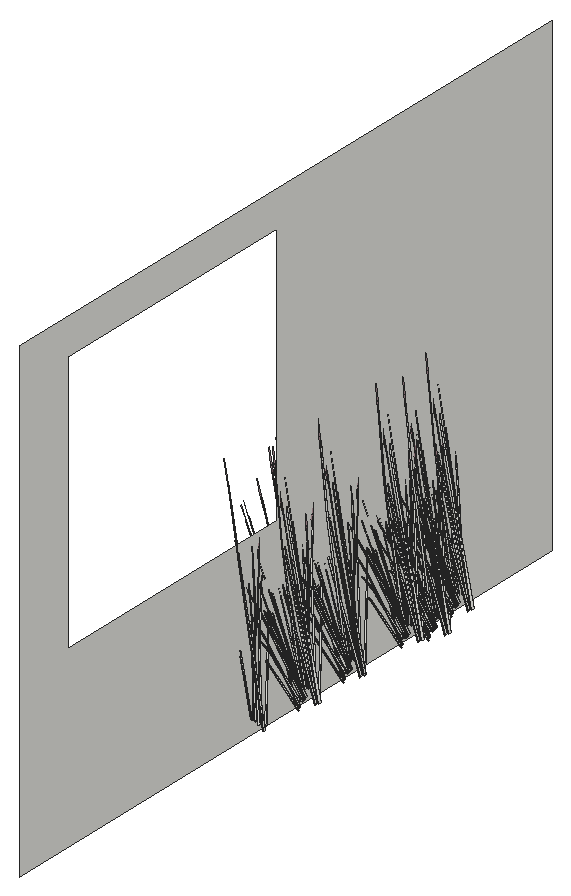
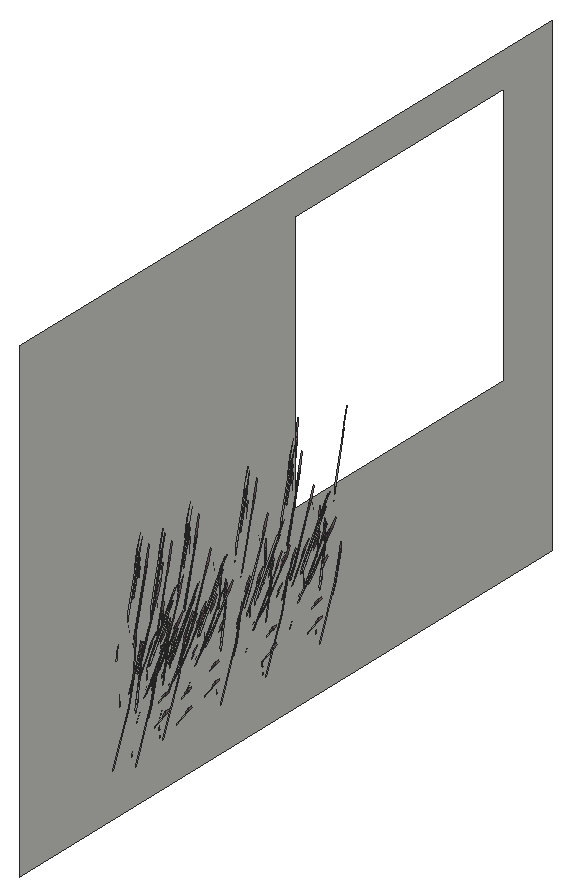
# SketchUp Ruby script. Lengths in inches.
U = 1.inch
M = Sketchup.active_model
def pt(a) = Geom::Point3d.new(a.map { |v| v * U })
def face(e, loops, mat)
  f = e.add_face(loops[0].map { |a| pt(a) })
  loops[1..].each { |l| e.add_face(l.map { |a| pt(a) }).erase! }
  f.material = f.back_material = mat if mat
  f
end
# faces: each face lists its corners as indices into pts; further lists are holes
def faces(e, pts, list, mat = nil) = list.each { |f| face(e, (f[0].is_a?(Array) ? f : [f]).map { |l| l.map { |i| pts[i] } }, mat) }
# xy, xz, yz: faces in a plane at the given z, y or x. An outline is a flat list of corners, or four numbers for a rectangle; further outlines are holes
def ring(l) = l.size == 4 ? [[l[0], l[1]], [l[2], l[1]], [l[2], l[3]], [l[0], l[3]]] : l.each_slice(2).to_a
def flat(e, list, mat, &to3) = list.each { |f| face(e, (f[0].is_a?(Array) ? f : [f]).map { |l| ring(l).map { |u, v| to3.(u, v) } }, mat) }
def xy(e, z, list, mat = nil) = flat(e, list, mat) { |x, y| [x, y, z] }
def xz(e, y, list, mat = nil) = flat(e, list, mat) { |x, z| [x, y, z] }
def yz(e, x, list, mat = nil) = flat(e, list, mat) { |y, z| [x, y, z] }
def lines(e, pts, list) = list.each { |a, b| e.add_line(pt(pts[a]), pt(pts[b])) }
# prism: a flat outline (further loops are holes) pulled along v
def prism(e, loops, v, mat = nil)
  f = face(e, loops, mat); d = Geom::Vector3d.new(v.map { |x| x * U })
  f.pushpull(f.normal.samedirection?(d) ? d.length : -d.length)
end
def box(e, o, s, mat = nil) = prism(e, [[o, [o[0] + s[0], o[1], o[2]], [o[0] + s[0], o[1] + s[1], o[2]], [o[0], o[1] + s[1], o[2]]]], [0, 0, s[2]], mat)
def at(x, y, z, deg = 0) = Geom::Transformation.translation(pt([x, y, z])) * Geom::Transformation.rotation(ORIGIN, Z_AXIS, deg.degrees)
def axes(o, x, y, z) = Geom::Transformation.new([*x, 0, *y, 0, *z, 0, *pt(o).to_a, 1])
def part(name) = M.definitions.add(name)
# library, detail: a bought-in or finely detailed component or shape, given as its bounding box
def library(name, o, s) = part(name).tap { |d| box(d.entities, o, s) }
def detail(e, o, s) = box(e.add_group.entities, o, s)
def put(e, d, t, mat = nil) = e.add_instance(d, t).tap { |i| i.material = mat if mat }
def group(e, t, mat = nil) = e.add_group.tap { |g| g.transformation = t; g.material = mat if mat }.entities
root = M.entities
M.materials.add("LightPink_Translucent").color = [144, 107, 117]
M.materials["LightPink_Translucent"].alpha = 0.75
c1 = part("blade")
p = [[2.15,0.21,22],[0,0.17,0],[0.09,0.45,0],[2.18,0.31,22],[2.29,0.31,22],[0.38,0.45,0],
  [2.48,0.24,33],[2.49,0.24,33],[2.48,0.22,33]]
faces(c1.entities,p,[[0,1,2,3],[4,5,2,3],[6,3,4,7],[8,0,3,6]])
c2 = part("seeds")
p = [[0.3,-0.1,1.38],[-0.01,-0.03,1.59],[-0.01,-0.03,0.03],[0.14,-0.07,-0.07],[0.29,-0.03,3],[0.15,0.01,3.11]]
faces(c2.entities,p,[[0,1,2,3],[1,0,4,5]],"LightPink_Translucent")
c3 = part("blade with seeds")
put(c3.entities,c1,at(0,0,0))
put(c3.entities,c2,axes([2.4,0.25,30.99],[1.5799,-0.05474,1.17369],[-0.12525,1.92788,0.29478],[-0.07173,-0.02425,1.56792]))
yz(root,336,[[[51,0,219,120],[66,45,132,111]]])
put(root,c3,axes([342.4,120.54,4.67],[-0.55932,0.6538,0],[-0.93577,-0.36461,-0.51607],[-0.21313,-0.08304,1.63711]))
put(root,c3,axes([340.23,119.03,7.02],[-0.61415,-0.2744,0.0643],[0.35756,-0.39076,0.50621],[-0.1969,0.12633,0.77189]))
put(root,c3,axes([340.93,118.95,7.34],[0.77872,-0.09325,0.35414],[0.20563,0.53305,-0.4572],[-0.22316,0.14318,0.87481]))
put(root,c3,axes([339.17,120.46,7.9375],[0.78943,0.17416,-0.06488],[-0.24284,0.53604,-0.29416],[-0.12912,0.08139,0.97024]))
put(root,c3,axes([340.53,118.9,7.33],[0.82753,0.35977,-0.1216],[-0.47675,0.52101,-0.67495],[-0.2338,0.18111,1.02557]))
put(root,c3,axes([340.94,119.32,6.97],[0.22982,0.59576,-0.51099],[-0.87033,0.10422,-0.3958],[-0.24941,0.16002,0.97773]))
put(root,c3,axes([341.4375,120.32,7.02],[-0.73517,-0.0304,0.0643],[0.02016,-0.45906,0.50621],[-0.07693,0.17585,0.77189]))
put(root,c3,axes([341.67,120.36,7.03],[-0.63704,-0.44518,0.48003],[0.67652,-0.38394,0.3958],[-0.11751,0.20886,0.9933]))
put(root,c3,axes([341.48,119.23,6.17],[0.16657,-0.22426,1.71376],[0.69879,0.4641,0.13857],[-0.31524,0.28926,0.73262]))
put(root,c3,axes([339.58,120.39,7.01],[-0.02224,0.12912,1.74944],[0.63107,0.44917,-0.27667],[-0.16521,0.21241,0.14031]))
put(root,c3,axes([341.38,121.49,4.88],[0.28231,-0.10293,1.43002],[0.69701,0.31035,-0.30754],[-0.20746,0.26854,0.61141]))
put(root,c3,axes([342.42,132.4375,6.17],[0.2045,0.20949,1.71376],[-0.94495,0.17636,0.13857],[-0.21357,-0.32887,0.73262]))
put(root,c3,axes([342.16,131.88,4.88],[-0.05417,0.21344,1.43002],[-0.79196,0.17867,-0.30754],[-0.18512,-0.27588,0.61141]))
put(root,c3,axes([343.05,130.75,7],[-0.01669,0.07821,1.77383],[-0.82314,0.28383,-0.16761],[-0.24223,-0.14508,0.31391]))
put(root,c3,axes([343.02,132.74,7.27],[-0.76283,-0.31537,-0.71045],[0.54213,-0.55263,0.08574],[-0.27638,-0.1883,1.00501]))
put(root,c3,axes([342.75,132.33,6.82],[-0.13817,-0.52554,-0.35414],[0.78985,-0.13877,0.4572],[-0.21215,-0.1506,0.87481]))
put(root,c3,axes([341.52,132.23,3.79],[-0.08666,0.08595,1.76342],[-0.87574,0.18531,-0.26939],[-0.21156,-0.16858,0.30037]))
put(root,c3,axes([342.66,132.76,6.97],[-0.88277,0.1551,-0.51099],[-0.15442,-0.58737,-0.3958],[-0.23711,-0.16832,0.97773]))
put(root,c3,axes([343.28,132.24,7.72],[-0.59706,0.6255,-0.13619],[-0.86465,-0.36036,-0.75594],[-0.30056,-0.17672,1.14864]))
put(root,c3,axes([340.85,133.1,7.39],[0.7388,-0.48151,0.53763],[0.63717,0.51135,0.4433],[-0.34662,-0.08882,1.11249]))
put(root,c3,axes([341.19,133.1,7.02],[0.04505,-0.49615,0.0643],[0.68022,0.0136,0.50621],[-0.26056,-0.05192,0.77189]))
put(root,c3,axes([340.98,132.56,4.42],[-0.25807,0.53277,-0.03893],[-0.79428,-0.16389,-0.17649],[-0.1206,-0.08714,0.58215]))
put(root,c3,axes([340.55,134.99,4.67],[-1.11865,0,0],[0,-0.72922,-0.51607],[0,-0.16609,1.63711]))
put(root,c3,axes([341.65,133.47,7.34],[0.50902,0.40851,0.35414],[-0.58122,0.38671,-0.4572],[-0.29531,-0.05884,0.87481]))
put(root,c3,axes([343.11,135.84,4.35],[-0.9306,-0.10697,-0.62353],[0.19638,-0.65984,-0.16365],[-0.27771,-0.07995,1.37633]))
put(root,c3,axes([342.12,136.84,4.32],[-0.21015,-0.56852,-0.30978],[0.83462,-0.16144,0.30978],[-0.16826,-0.06556,1.38974]))
put(root,c3,axes([341.89,137.08,4.3125],[-0.83726,-0.32623,-0.49651],[0.50045,-0.58498,0],[-0.19069,-0.0743,1.57504]))
put(root,c3,axes([344.17,135.93,4.96],[-0.90324,0.43318,-0.29095],[-0.60064,-0.61207,-0.50002],[-0.22285,-0.06216,1.59708]))
put(root,c3,axes([340.81,134.61,7.34],[0.74348,0.18202,0.35414],[-0.21685,0.53102,-0.4572],[-0.29933,0.04869,0.87481]))
put(root,c3,axes([342.4,137.48,4.67],[-0.55932,0.6538,0],[-0.93577,-0.36461,-0.51607],[-0.21313,-0.08304,1.63711]))
put(root,c3,axes([340.23,135.97,7.02],[-0.61415,-0.2744,0.0643],[0.35756,-0.39076,0.50621],[-0.1969,0.12633,0.77189]))
put(root,c3,axes([340.93,135.89,7.34],[0.77872,-0.09325,0.35414],[0.20563,0.53305,-0.4572],[-0.22316,0.14318,0.87481]))
put(root,c3,axes([339.17,137.4,7.9375],[0.78943,0.17416,-0.06488],[-0.24284,0.53604,-0.29416],[-0.12912,0.08139,0.97024]))
put(root,c3,axes([340.53,135.84,7.33],[0.82753,0.35977,-0.1216],[-0.47675,0.52101,-0.67495],[-0.2338,0.18111,1.02557]))
put(root,c3,axes([340.94,136.26,6.97],[0.22982,0.59576,-0.51099],[-0.87033,0.10422,-0.3958],[-0.24941,0.16002,0.97773]))
put(root,c3,axes([341.67,137.3,7.03],[-0.63704,-0.44518,0.48003],[0.67652,-0.38394,0.3958],[-0.11751,0.20886,0.9933]))
put(root,c3,axes([342.42,146.79,6.17],[0.2045,0.20949,1.71376],[-0.94495,0.17636,0.13857],[-0.21357,-0.32887,0.73262]))
put(root,c3,axes([341.48,136.17,6.17],[0.16657,-0.22426,1.71376],[0.69879,0.4641,0.13857],[-0.31524,0.28926,0.73262]))
put(root,c3,axes([339.58,137.33,7.01],[-0.02224,0.12912,1.74944],[0.63107,0.44917,-0.27667],[-0.16521,0.21241,0.14031]))
put(root,c3,axes([342.16,146.23,4.88],[-0.05417,0.21344,1.43002],[-0.79196,0.17867,-0.30754],[-0.18512,-0.27588,0.61141]))
put(root,c3,axes([343.05,145.1,7],[-0.01669,0.07821,1.77383],[-0.82314,0.28383,-0.16761],[-0.24223,-0.14508,0.31391]))
put(root,c3,axes([343.02,147.09,7.27],[-0.76283,-0.31537,-0.71045],[0.54213,-0.55263,0.08574],[-0.27638,-0.1883,1.00501]))
put(root,c3,axes([342.75,146.67,6.82],[-0.13817,-0.52554,-0.35414],[0.78985,-0.13877,0.4572],[-0.21215,-0.1506,0.87481]))
put(root,c3,axes([341.38,138.43,4.88],[0.28231,-0.10293,1.43002],[0.69701,0.31035,-0.30754],[-0.20746,0.26854,0.61141]))
put(root,c3,axes([341.52,146.57,3.79],[-0.08666,0.08595,1.76342],[-0.87574,0.18531,-0.26939],[-0.21156,-0.16858,0.30037]))
put(root,c3,axes([342.66,147.11,6.97],[-0.88277,0.1551,-0.51099],[-0.15442,-0.58737,-0.3958],[-0.23711,-0.16832,0.97773]))
put(root,c3,axes([343.28,146.58,7.72],[-0.59706,0.6255,-0.13619],[-0.86465,-0.36036,-0.75594],[-0.30056,-0.17672,1.14864]))
put(root,c3,axes([340.85,147.45,7.39],[0.7388,-0.48151,0.53763],[0.63717,0.51135,0.4433],[-0.34662,-0.08882,1.11249]))
put(root,c3,axes([341.19,147.44,7.02],[0.04505,-0.49615,0.0643],[0.68022,0.0136,0.50621],[-0.26056,-0.05192,0.77189]))
put(root,c3,axes([340.98,146.9,4.42],[-0.25807,0.53277,-0.03893],[-0.79428,-0.16389,-0.17649],[-0.1206,-0.08714,0.58215]))
put(root,c3,axes([340.55,149.34,4.67],[-1.11865,0,0],[0,-0.72922,-0.51607],[0,-0.16609,1.63711]))
put(root,c3,axes([341.65,147.8125,7.34],[0.50902,0.40851,0.35414],[-0.58122,0.38671,-0.4572],[-0.29531,-0.05884,0.87481]))
put(root,c3,axes([343.11,150.18,4.35],[-0.9306,-0.10697,-0.62353],[0.19638,-0.65984,-0.16365],[-0.27771,-0.07995,1.37633]))
put(root,c3,axes([342.12,151.1875,4.32],[-0.21015,-0.56852,-0.30978],[0.83462,-0.16144,0.30978],[-0.16826,-0.06556,1.38974]))
put(root,c3,axes([341.89,151.43,4.3125],[-0.83726,-0.32623,-0.49651],[0.50045,-0.58498,0],[-0.19069,-0.0743,1.57504]))
put(root,c3,axes([344.17,150.28,4.96],[-0.90324,0.43318,-0.29095],[-0.60064,-0.61207,-0.50002],[-0.22285,-0.06216,1.59708]))
put(root,c3,axes([340.81,148.96,7.34],[0.74348,0.18202,0.35414],[-0.21685,0.53102,-0.4572],[-0.29933,0.04869,0.87481]))
put(root,c3,axes([342.4,151.83,4.67],[-0.55932,0.6538,0],[-0.93577,-0.36461,-0.51607],[-0.21313,-0.08304,1.63711]))
put(root,c3,axes([340.23,150.32,7.02],[-0.61415,-0.2744,0.0643],[0.35756,-0.39076,0.50621],[-0.1969,0.12633,0.77189]))
put(root,c3,axes([340.93,150.23,7.34],[0.77872,-0.09325,0.35414],[0.20563,0.53305,-0.4572],[-0.22316,0.14318,0.87481]))
put(root,c3,axes([339.17,151.75,7.9375],[0.78943,0.17416,-0.06488],[-0.24284,0.53604,-0.29416],[-0.12912,0.08139,0.97024]))
put(root,c3,axes([340.53,150.18,7.33],[0.82753,0.35977,-0.1216],[-0.47675,0.52101,-0.67495],[-0.2338,0.18111,1.02557]))
put(root,c3,axes([340.94,150.61,6.97],[0.22982,0.59576,-0.51099],[-0.87033,0.10422,-0.3958],[-0.24941,0.16002,0.97773]))
put(root,c3,axes([341.67,151.65,7.03],[-0.63704,-0.44518,0.48003],[0.67652,-0.38394,0.3958],[-0.11751,0.20886,0.9933]))
put(root,c3,axes([341.48,150.52,6.17],[0.16657,-0.22426,1.71376],[0.69879,0.4641,0.13857],[-0.31524,0.28926,0.73262]))
put(root,c3,axes([339.58,151.68,7.01],[-0.02224,0.12912,1.74944],[0.63107,0.44917,-0.27667],[-0.16521,0.21241,0.14031]))
put(root,c3,axes([341.38,152.77,4.88],[0.28231,-0.10293,1.43002],[0.69701,0.31035,-0.30754],[-0.20746,0.26854,0.61141]))
put(root,c3,axes([342.42,164.95,6.17],[0.2045,0.20949,1.71376],[-0.94495,0.17636,0.13857],[-0.21357,-0.32887,0.73262]))
put(root,c3,axes([342.16,164.4,4.88],[-0.05417,0.21344,1.43002],[-0.79196,0.17867,-0.30754],[-0.18512,-0.27588,0.61141]))
put(root,c3,axes([343.05,163.26,7],[-0.01669,0.07821,1.77383],[-0.82314,0.28383,-0.16761],[-0.24223,-0.14508,0.31391]))
put(root,c3,axes([343.02,165.26,7.27],[-0.76283,-0.31537,-0.71045],[0.54213,-0.55263,0.08574],[-0.27638,-0.1883,1.00501]))
put(root,c3,axes([342.75,164.84,6.82],[-0.13817,-0.52554,-0.35414],[0.78985,-0.13877,0.4572],[-0.21215,-0.1506,0.87481]))
put(root,c3,axes([341.52,164.74,3.79],[-0.08666,0.08595,1.76342],[-0.87574,0.18531,-0.26939],[-0.21156,-0.16858,0.30037]))
put(root,c3,axes([342.66,165.27,6.97],[-0.88277,0.1551,-0.51099],[-0.15442,-0.58737,-0.3958],[-0.23711,-0.16832,0.97773]))
put(root,c3,axes([343.28,164.75,7.72],[-0.59706,0.6255,-0.13619],[-0.86465,-0.36036,-0.75594],[-0.30056,-0.17672,1.14864]))
put(root,c3,axes([340.85,165.61,7.39],[0.7388,-0.48151,0.53763],[0.63717,0.51135,0.4433],[-0.34662,-0.08882,1.11249]))
put(root,c3,axes([341.19,165.61,7.02],[0.04505,-0.49615,0.0643],[0.68022,0.0136,0.50621],[-0.26056,-0.05192,0.77189]))
put(root,c3,axes([340.98,165.07,4.42],[-0.25807,0.53277,-0.03893],[-0.79428,-0.16389,-0.17649],[-0.1206,-0.08714,0.58215]))
put(root,c3,axes([340.55,167.5,4.67],[-1.11865,0,0],[0,-0.72922,-0.51607],[0,-0.16609,1.63711]))
put(root,c3,axes([341.65,165.98,7.34],[0.50902,0.40851,0.35414],[-0.58122,0.38671,-0.4572],[-0.29531,-0.05884,0.87481]))
put(root,c3,axes([343.11,168.35,4.35],[-0.9306,-0.10697,-0.62353],[0.19638,-0.65984,-0.16365],[-0.27771,-0.07995,1.37633]))
put(root,c3,axes([342.12,169.35,4.32],[-0.21015,-0.56852,-0.30978],[0.83462,-0.16144,0.30978],[-0.16826,-0.06556,1.38974]))
put(root,c3,axes([341.89,169.6,4.3125],[-0.83726,-0.32623,-0.49651],[0.50045,-0.58498,0],[-0.19069,-0.0743,1.57504]))
put(root,c3,axes([344.17,168.45,4.96],[-0.90324,0.43318,-0.29095],[-0.60064,-0.61207,-0.50002],[-0.22285,-0.06216,1.59708]))
put(root,c3,axes([342.42,173.6,3.875],[0.2045,0.20949,1.71376],[-0.94495,0.17636,0.13857],[-0.21357,-0.32887,0.73262]))
put(root,c3,axes([340.81,167.12,7.34],[0.74348,0.18202,0.35414],[-0.21685,0.53102,-0.4572],[-0.29933,0.04869,0.87481]))
put(root,c3,axes([342.16,173.05,2.59],[-0.05417,0.21344,1.43002],[-0.79196,0.17867,-0.30754],[-0.18512,-0.27588,0.61141]))
put(root,c3,axes([342.4,169.99,4.67],[-0.55932,0.6538,0],[-0.93577,-0.36461,-0.51607],[-0.21313,-0.08304,1.63711]))
put(root,c3,axes([343.05,171.91,4.71],[-0.01669,0.07821,1.77383],[-0.82314,0.28383,-0.16761],[-0.24223,-0.14508,0.31391]))
put(root,c3,axes([343.02,173.91,4.98],[-0.76283,-0.31537,-0.71045],[0.54213,-0.55263,0.08574],[-0.27638,-0.1883,1.00501]))
put(root,c3,axes([342.75,173.49,4.53],[-0.13817,-0.52554,-0.35414],[0.78985,-0.13877,0.4572],[-0.21215,-0.1506,0.87481]))
put(root,c3,axes([340.23,168.48,7.02],[-0.61415,-0.2744,0.0643],[0.35756,-0.39076,0.50621],[-0.1969,0.12633,0.77189]))
put(root,c3,axes([341.52,173.39,1.49],[-0.08666,0.08595,1.76342],[-0.87574,0.18531,-0.26939],[-0.21156,-0.16858,0.30037]))
put(root,c3,axes([340.93,168.4,7.34],[0.77872,-0.09325,0.35414],[0.20563,0.53305,-0.4572],[-0.22316,0.14318,0.87481]))
put(root,c3,axes([342.66,173.93,4.68],[-0.88277,0.1551,-0.51099],[-0.15442,-0.58737,-0.3958],[-0.23711,-0.16832,0.97773]))
put(root,c3,axes([343.28,173.4,5.43],[-0.59706,0.6255,-0.13619],[-0.86465,-0.36036,-0.75594],[-0.30056,-0.17672,1.14864]))
put(root,c3,axes([339.17,169.91,7.9375],[0.78943,0.17416,-0.06488],[-0.24284,0.53604,-0.29416],[-0.12912,0.08139,0.97024]))
put(root,c3,axes([340.85,174.26,5.09],[0.7388,-0.48151,0.53763],[0.63717,0.51135,0.4433],[-0.34662,-0.08882,1.11249]))
put(root,c3,axes([340.53,168.35,7.33],[0.82753,0.35977,-0.1216],[-0.47675,0.52101,-0.67495],[-0.2338,0.18111,1.02557]))
put(root,c3,axes([340.94,168.78,6.97],[0.22982,0.59576,-0.51099],[-0.87033,0.10422,-0.3958],[-0.24941,0.16002,0.97773]))
put(root,c3,axes([341.19,174.26,4.73],[0.04505,-0.49615,0.0643],[0.68022,0.0136,0.50621],[-0.26056,-0.05192,0.77189]))
put(root,c3,axes([341.67,169.8125,7.03],[-0.63704,-0.44518,0.48003],[0.67652,-0.38394,0.3958],[-0.11751,0.20886,0.9933]))
put(root,c3,axes([340.98,173.72,2.13],[-0.25807,0.53277,-0.03893],[-0.79428,-0.16389,-0.17649],[-0.1206,-0.08714,0.58215]))
put(root,c3,axes([340.55,176.15,2.375],[-1.11865,0,0],[0,-0.72922,-0.51607],[0,-0.16609,1.63711]))
put(root,c3,axes([341.48,168.68,6.17],[0.16657,-0.22426,1.71376],[0.69879,0.4641,0.13857],[-0.31524,0.28926,0.73262]))
put(root,c3,axes([339.58,169.85,7.01],[-0.02224,0.12912,1.74944],[0.63107,0.44917,-0.27667],[-0.16521,0.21241,0.14031]))
put(root,c3,axes([341.65,174.63,5.05],[0.50902,0.40851,0.35414],[-0.58122,0.38671,-0.4572],[-0.29531,-0.05884,0.87481]))
put(root,c3,axes([342.42,180.77,6.17],[0.2045,0.20949,1.71376],[-0.94495,0.17636,0.13857],[-0.21357,-0.32887,0.73262]))
put(root,c3,axes([343.11,177,2.06],[-0.9306,-0.10697,-0.62353],[0.19638,-0.65984,-0.16365],[-0.27771,-0.07995,1.37633]))
put(root,c3,axes([342.16,180.22,4.88],[-0.05417,0.21344,1.43002],[-0.79196,0.17867,-0.30754],[-0.18512,-0.27588,0.61141]))
put(root,c3,axes([341.38,170.9375,4.88],[0.28231,-0.10293,1.43002],[0.69701,0.31035,-0.30754],[-0.20746,0.26854,0.61141]))
put(root,c3,axes([342.12,178.01,2.03],[-0.21015,-0.56852,-0.30978],[0.83462,-0.16144,0.30978],[-0.16826,-0.06556,1.38974]))
put(root,c3,axes([341.89,178.25,2.02],[-0.83726,-0.32623,-0.49651],[0.50045,-0.58498,0],[-0.19069,-0.0743,1.57504]))
put(root,c3,axes([344.17,177.1,2.67],[-0.90324,0.43318,-0.29095],[-0.60064,-0.61207,-0.50002],[-0.22285,-0.06216,1.59708]))
put(root,c3,axes([343.05,179.08,7],[-0.01669,0.07821,1.77383],[-0.82314,0.28383,-0.16761],[-0.24223,-0.14508,0.31391]))
put(root,c3,axes([340.81,175.78,5.05],[0.74348,0.18202,0.35414],[-0.21685,0.53102,-0.4572],[-0.29933,0.04869,0.87481]))
put(root,c3,axes([343.02,181.08,7.27],[-0.76283,-0.31537,-0.71045],[0.54213,-0.55263,0.08574],[-0.27638,-0.1883,1.00501]))
put(root,c3,axes([342.75,180.66,6.82],[-0.13817,-0.52554,-0.35414],[0.78985,-0.13877,0.4572],[-0.21215,-0.1506,0.87481]))
put(root,c3,axes([341.52,180.56,3.79],[-0.08666,0.08595,1.76342],[-0.87574,0.18531,-0.26939],[-0.21156,-0.16858,0.30037]))
put(root,c3,axes([342.4,178.64,2.375],[-0.55932,0.6538,0],[-0.93577,-0.36461,-0.51607],[-0.21313,-0.08304,1.63711]))
put(root,c3,axes([342.66,181.09,6.97],[-0.88277,0.1551,-0.51099],[-0.15442,-0.58737,-0.3958],[-0.23711,-0.16832,0.97773]))
put(root,c3,axes([343.28,180.57,7.72],[-0.59706,0.6255,-0.13619],[-0.86465,-0.36036,-0.75594],[-0.30056,-0.17672,1.14864]))
put(root,c3,axes([340.23,177.14,4.73],[-0.61415,-0.2744,0.0643],[0.35756,-0.39076,0.50621],[-0.1969,0.12633,0.77189]))
put(root,c3,axes([340.85,181.43,7.39],[0.7388,-0.48151,0.53763],[0.63717,0.51135,0.4433],[-0.34662,-0.08882,1.11249]))
put(root,c3,axes([340.93,177.05,5.05],[0.77872,-0.09325,0.35414],[0.20563,0.53305,-0.4572],[-0.22316,0.14318,0.87481]))
put(root,c3,axes([341.19,181.43,7.02],[0.04505,-0.49615,0.0643],[0.68022,0.0136,0.50621],[-0.26056,-0.05192,0.77189]))
put(root,c3,axes([340.98,180.89,4.42],[-0.25807,0.53277,-0.03893],[-0.79428,-0.16389,-0.17649],[-0.1206,-0.08714,0.58215]))
put(root,c3,axes([340.55,183.32,4.67],[-1.11865,0,0],[0,-0.72922,-0.51607],[0,-0.16609,1.63711]))
put(root,c3,axes([339.17,178.56,5.65],[0.78943,0.17416,-0.06488],[-0.24284,0.53604,-0.29416],[-0.12912,0.08139,0.97024]))
put(root,c3,axes([340.53,177,5.03],[0.82753,0.35977,-0.1216],[-0.47675,0.52101,-0.67495],[-0.2338,0.18111,1.02557]))
put(root,c3,axes([340.94,177.43,4.68],[0.22982,0.59576,-0.51099],[-0.87033,0.10422,-0.3958],[-0.24941,0.16002,0.97773]))
put(root,c3,axes([341.65,181.8,7.34],[0.50902,0.40851,0.35414],[-0.58122,0.38671,-0.4572],[-0.29531,-0.05884,0.87481]))
put(root,c3,axes([341.67,178.47,4.73],[-0.63704,-0.44518,0.48003],[0.67652,-0.38394,0.3958],[-0.11751,0.20886,0.9933]))
put(root,c3,axes([341.48,177.34,3.875],[0.16657,-0.22426,1.71376],[0.69879,0.4641,0.13857],[-0.31524,0.28926,0.73262]))
put(root,c3,axes([343.11,184.17,4.35],[-0.9306,-0.10697,-0.62353],[0.19638,-0.65984,-0.16365],[-0.27771,-0.07995,1.37633]))
put(root,c3,axes([339.58,178.5,4.72],[-0.02224,0.12912,1.74944],[0.63107,0.44917,-0.27667],[-0.16521,0.21241,0.14031]))
put(root,c3,axes([342.12,185.17,4.32],[-0.21015,-0.56852,-0.30978],[0.83462,-0.16144,0.30978],[-0.16826,-0.06556,1.38974]))
put(root,c3,axes([341.89,185.42,4.3125],[-0.83726,-0.32623,-0.49651],[0.50045,-0.58498,0],[-0.19069,-0.0743,1.57504]))
put(root,c3,axes([344.17,184.27,4.96],[-0.90324,0.43318,-0.29095],[-0.60064,-0.61207,-0.50002],[-0.22285,-0.06216,1.59708]))
put(root,c3,axes([340.81,182.94,7.34],[0.74348,0.18202,0.35414],[-0.21685,0.53102,-0.4572],[-0.29933,0.04869,0.87481]))
put(root,c3,axes([341.38,179.59,2.59],[0.28231,-0.10293,1.43002],[0.69701,0.31035,-0.30754],[-0.20746,0.26854,0.61141]))
put(root,c3,axes([342.4,185.8125,4.67],[-0.55932,0.6538,0],[-0.93577,-0.36461,-0.51607],[-0.21313,-0.08304,1.63711]))
put(root,c3,axes([340.23,184.3,7.02],[-0.61415,-0.2744,0.0643],[0.35756,-0.39076,0.50621],[-0.1969,0.12633,0.77189]))
put(root,c3,axes([340.93,184.22,7.34],[0.77872,-0.09325,0.35414],[0.20563,0.53305,-0.4572],[-0.22316,0.14318,0.87481]))
